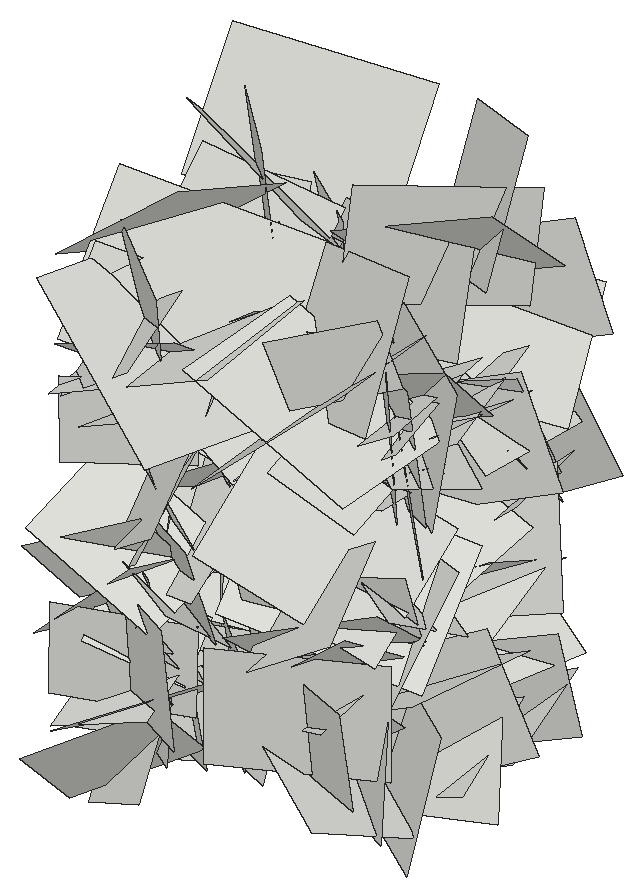
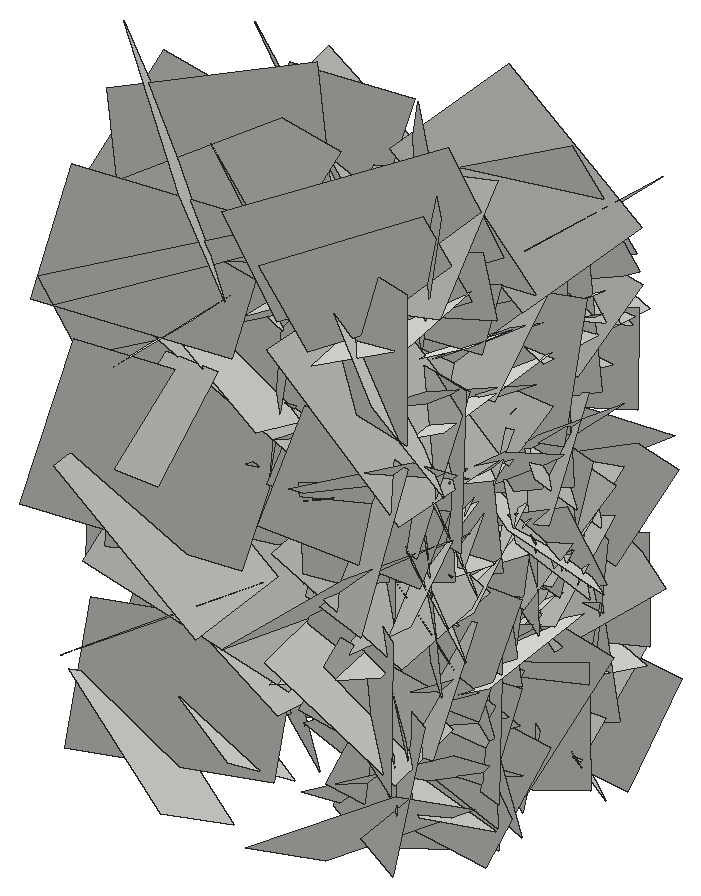
# SketchUp Ruby script. Lengths in inches.
U = 1.inch
M = Sketchup.active_model
def pt(a) = Geom::Point3d.new(a.map { |v| v * U })
def face(e, loops, mat)
  f = e.add_face(loops[0].map { |a| pt(a) })
  loops[1..].each { |l| e.add_face(l.map { |a| pt(a) }).erase! }
  f.material = f.back_material = mat if mat
  f
end
# faces: each face lists its corners as indices into pts; further lists are holes
def faces(e, pts, list, mat = nil) = list.each { |f| face(e, (f[0].is_a?(Array) ? f : [f]).map { |l| l.map { |i| pts[i] } }, mat) }
# xy, xz, yz: faces in a plane at the given z, y or x. An outline is a flat list of corners, or four numbers for a rectangle; further outlines are holes
def ring(l) = l.size == 4 ? [[l[0], l[1]], [l[2], l[1]], [l[2], l[3]], [l[0], l[3]]] : l.each_slice(2).to_a
def flat(e, list, mat, &to3) = list.each { |f| face(e, (f[0].is_a?(Array) ? f : [f]).map { |l| ring(l).map { |u, v| to3.(u, v) } }, mat) }
def xy(e, z, list, mat = nil) = flat(e, list, mat) { |x, y| [x, y, z] }
def xz(e, y, list, mat = nil) = flat(e, list, mat) { |x, z| [x, y, z] }
def yz(e, x, list, mat = nil) = flat(e, list, mat) { |y, z| [x, y, z] }
def lines(e, pts, list) = list.each { |a, b| e.add_line(pt(pts[a]), pt(pts[b])) }
# prism: a flat outline (further loops are holes) pulled along v
def prism(e, loops, v, mat = nil)
  f = face(e, loops, mat); d = Geom::Vector3d.new(v.map { |x| x * U })
  f.pushpull(f.normal.samedirection?(d) ? d.length : -d.length)
end
def box(e, o, s, mat = nil) = prism(e, [[o, [o[0] + s[0], o[1], o[2]], [o[0] + s[0], o[1] + s[1], o[2]], [o[0], o[1] + s[1], o[2]]]], [0, 0, s[2]], mat)
def at(x, y, z, deg = 0) = Geom::Transformation.translation(pt([x, y, z])) * Geom::Transformation.rotation(ORIGIN, Z_AXIS, deg.degrees)
def axes(o, x, y, z) = Geom::Transformation.new([*x, 0, *y, 0, *z, 0, *pt(o).to_a, 1])
def part(name) = M.definitions.add(name)
# library, detail: a bought-in or finely detailed component or shape, given as its bounding box
def library(name, o, s) = part(name).tap { |d| box(d.entities, o, s) }
def detail(e, o, s) = box(e.add_group.entities, o, s)
def put(e, d, t, mat = nil) = e.add_instance(d, t).tap { |i| i.material = mat if mat }
def group(e, t, mat = nil) = e.add_group.tap { |g| g.transformation = t; g.material = mat if mat }.entities
root = M.entities
c1 = part("Component\#6")
p = [[0.01,0,0],[0,3.24,4.54],[4.32,3.24,4.54],[4.33,0,0]]
faces(c1.entities,p,[[0,1,2,3]])
put(root,c1,axes([414.68,154.27,5.56],[0.10843,0.64197,-0.78685],[0.13439,-0.79271,-0.63027],[-1.06801,-0.03458,-0.15919]))
put(root,c1,axes([410.71,149.67,1.32],[0.10197,-0.47157,-0.58691],[-0.00963,-0.59236,0.47447],[0.798,0.05311,0.08072]))
put(root,c1,axes([410.71,151.77,10.3],[0.00621,-0.04081,-0.81439],[0.02737,-0.814,0.04098],[0.86391,0.02608,0.00455]))
put(root,c1,axes([414.68,158.76,13.54],[0.17018,-0.33172,-0.9968],[0.1229,-0.99662,0.35033],[-1.10678,-0.16167,-0.11436]))
put(root,c1,axes([410.71,155.14,21.07],[-0.01676,0.7943,-0.14622],[0.08914,-0.14383,-0.79043],[0.85145,0.03069,0.07988]))
put(root,c1,axes([414.68,152.55,8.85],[0.17208,0.39932,0.93109],[0.08126,0.93542,-0.41455],[-1.07081,0.13515,0.11817]))
put(root,c1,axes([410.71,155.22,14.18],[-0.0107,0.67836,0.43703],[0.08223,0.43585,-0.67474],[0.8514,-0.03357,0.07066]))
put(root,c1,axes([414.68,154.72,7.86],[-0.01434,-0.12328,-0.7123],[-0.10241,-0.70572,0.12398],[-0.75939,0.0975,-0.00327]))
put(root,c1,axes([410.71,153.88,7.81],[0.12498,-0.19712,-0.75186],[-0.05107,-0.76085,0.19192],[0.82232,-0.01729,0.12619]))
put(root,c1,axes([414.68,156.49,11.61],[0.16435,-0.92659,-0.48849],[0.14398,-0.47186,0.93815],[-1.10094,-0.20004,0.04977]))
put(root,c1,axes([414.68,155.82,10.86],[0.10869,-0.77244,0.23734],[-0.13092,0.22145,0.77409],[-0.8465,-0.13343,-0.08925]))
put(root,c1,axes([410.71,152.8,10.75],[-0.04843,-0.82009,-0.82841],[-0.32646,-0.79109,0.80013],[1.19171,-0.25004,0.18553]))
put(root,c1,axes([410.71,146.53,12.92],[0.03124,-0.05121,0.8385],[-0.00373,0.839,0.05136],[0.89046,0.00531,-0.0292]))
put(root,c1,axes([410.71,155.95,10.68],[0.04823,-0.00518,0.84226],[-0.02844,0.84305,0.00663],[0.89236,0.02715,-0.04531]))
put(root,c1,axes([414.68,154.86,6.54],[0.11481,0.21277,-0.79232],[-0.09254,-0.79167,-0.22453],[-0.86468,0.11298,-0.08117]))
put(root,c1,axes([410.71,147.06,-0.97],[0.01135,-0.66277,0.66685],[-0.09721,0.66298,0.66039],[0.99185,0.07256,0.05709]))
put(root,c1,axes([414.68,155.74,21.65],[0.00825,-0.17983,-0.66547],[-0.14401,-0.65286,0.17483],[-0.71636,0.12918,-0.04281]))
put(root,c1,axes([414.68,153.02,6.56],[-0.04835,0.51462,-0.41299],[-0.10228,-0.41473,-0.50612],[-0.69191,0.02534,0.10368]))
put(root,c1,axes([410.71,149.625,17.57],[0.05592,-0.7816,-0.40589],[-0.0657,-0.4089,0.77935],[0.93124,0.01809,0.07936]))
put(root,c1,axes([410.71,152.46,19.1],[-0.24316,-1.11668,0.32256],[-0.08367,0.34299,1.13127],[1.22923,-0.19755,0.14081]))
put(root,c1,axes([410.71,154.93,13.48],[-0.13332,0.92748,-0.67904],[-0.1887,-0.69057,-0.91025],[1.20375,-0.00553,-0.2179]))
put(root,c1,axes([414.68,155.23,10.47],[0.04155,0.12694,-0.87349],[0.11983,-0.86787,-0.12105],[-0.92792,-0.10639,-0.05475]))
put(root,c1,axes([410.71,153.68,-0.24],[0.08313,-0.05331,0.78078],[0.05564,0.78328,0.04821],[0.82769,-0.0473,-0.08166]))
put(root,c1,axes([414.68,152.53,7.1875],[-0.08757,-0.64703,0.3684],[0.09594,0.35919,0.65114],[-0.78338,0.11632,0.03856]))
put(root,c1,axes([414.68,154.48,3.89],[-0.11783,0.23417,0.69133],[0.11259,0.69704,-0.21902],[-0.76547,0.06648,-0.13863]))
put(root,c1,axes([410.71,151.57,3.27],[0.14157,0.02397,-0.74069],[0.04702,-0.75154,-0.01632],[0.78414,0.04073,0.1347]))
put(root,c1,axes([414.68,146.09,12.1875],[0.18427,0.52878,-0.65011],[-0.11203,-0.64482,-0.55274],[-0.8812,0.19255,-0.06567]))
put(root,c1,axes([410.71,147.21,13.43],[-0.06341,1.09172,0.23851],[-0.19798,0.22572,-1.08003],[1.16785,0.09755,-0.17015]))
put(root,c1,axes([414.68,145.53,10.42],[0.22479,1.04725,-0.16356],[0.16331,-0.19548,-1.05191],[-1.11161,0.18306,-0.18761]))
put(root,c1,axes([410.71,149.03,14.67],[-0.12882,0.64149,-0.81464],[0.00451,-0.8199,-0.64626],[1.09909,0.07855,-0.09282]))
put(root,c1,axes([414.68,155.43,2.74],[-0.05213,0.12024,0.7107],[0.06472,0.71048,-0.11598],[-0.7613,0.05216,-0.05853]))
put(root,c1,axes([410.71,146.38,17.95],[0.09245,0.38694,0.78979],[-0.04684,0.79459,-0.38441],[0.93107,0.00155,-0.09776]))
put(root,c1,axes([414.68,155.07,5.6],[0.26442,-0.95782,0.42161],[0.12666,0.45666,0.96674],[-1.10204,-0.17733,0.21227]))
put(root,c1,axes([414.68,154.81,5.31],[-0.03271,-0.68931,-0.29186],[0.0897,-0.29345,0.68411],[-0.78838,-0.00479,0.08995]))
put(root,c1,axes([414.68,148.44,10.1],[-0.02371,0.59128,0.15103],[-0.13632,0.14317,-0.57956],[-0.63236,-0.05303,0.11928]))
put(root,c1,axes([410.71,154.73,4.99],[-0.23466,-0.21907,1.02966],[0.17179,1.03255,0.25453],[1.10257,-0.20751,0.17949]))
put(root,c1,axes([410.71,152.28,1.18],[-0.22482,-0.75958,0.923],[-0.06114,0.94282,0.76264],[1.2656,-0.08938,0.2008]))
put(root,c1,axes([414.68,146.72,8.375],[-0.05548,0.31048,0.67068],[0.12303,0.66747,-0.29994],[-0.77368,0.08387,-0.09579]))
put(root,c1,axes([410.71,147.71,9.53],[-0.0202,0.73421,-0.62443],[0.01239,-0.62433,-0.73445],[1.02159,0.02209,-0.00344]))
put(root,c1,axes([414.68,148.39,13.69],[-0.056,0.56116,0.2115],[-0.06403,0.20626,-0.56234],[-0.63244,-0.07057,0.03821]))
put(root,c1,axes([410.71,149.64,15.49],[-0.05397,-0.71515,0.49033],[0.26351,0.45852,0.69456],[0.88054,-0.18105,-0.1778]))
put(root,c1,axes([410.71,157.06,14.03],[-0.04606,-0.47436,-0.98882],[-0.12961,-0.98133,0.47614],[1.15527,-0.12901,0.01399]))
put(root,c1,axes([410.71,159.16,9.85],[-0.13765,0.1916,-1.18129],[-0.14512,-1.1828,-0.17679],[1.2602,-0.11528,-0.14939]))
put(root,c1,axes([410.71,152.91,14.99],[-0.05042,0.65822,-0.8803],[-0.11398,-0.87969,-0.65195],[1.15954,-0.05785,-0.10236]))
put(root,c1,axes([410.71,158.68,8.63],[-0.07829,-0.94373,0.27717],[0.10215,0.26967,0.94388],[1.03759,-0.09775,-0.07202]))
put(root,c1,axes([414.68,147.13,6.96],[0.04816,-0.19283,0.63159],[-0.07038,0.62854,0.19668],[-0.69645,-0.07685,0.0238]))
put(root,c1,axes([410.71,152.6,3.91],[0.02426,0.68313,0.69515],[-0.0107,0.69547,-0.68312],[1.03305,-0.00884,-0.0234]))
put(root,c1,axes([414.68,153.92,20.8125],[-0.01755,0.277,-0.54123],[-0.05617,-0.54003,-0.27476],[-0.64202,0.03967,0.03883]))
put(root,c1,axes([414.68,156.87,7.65],[-0.00449,0.50233,-0.39291],[-0.02578,-0.39276,-0.50188],[-0.67552,0.01165,0.02176]))
put(root,c1,axes([414.68,147.62,1.41],[0.08717,-0.06025,0.7019],[-0.04865,0.70471,0.06586],[-0.74517,-0.05306,0.07781]))
put(root,c1,axes([414.68,151.79,4.27],[0.00282,-0.67031,0.14172],[0.04158,0.14164,0.66918],[-0.72504,0.00552,0.03892]))
put(root,c1,axes([414.68,151.99,2.12],[0.1775,0.68354,0.35821],[-0.06031,0.37649,-0.69181],[-0.81579,0.12089,0.12909]))
put(root,c1,axes([410.71,154.79,8.7],[-0.06507,0.61236,-0.89404],[-0.03144,-0.89608,-0.61173],[1.14823,0.01016,-0.06741]))
put(root,c1,axes([410.71,155.05,20.66],[0.11898,0.43702,0.87755],[-0.10329,0.88388,-0.42771],[1.03402,0.038,-0.1437]))
put(root,c1,axes([410.71,148.76,4.0625],[0.10183,-0.75916,-0.2873],[0.20096,-0.26032,0.75126],[0.83661,0.15493,-0.14549]))
put(root,c1,axes([414.68,151.13,9.12],[0.15296,0.67587,0.31221],[-0.03502,0.32352,-0.68509],[-0.78839,0.11676,0.09101]))
put(root,c1,axes([410.71,158.45,22.43],[-0.19892,0.24365,-1.12098],[0.08242,-1.13056,-0.25875],[1.21318,0.11676,-0.16622]))
put(root,c1,axes([410.71,153.47,7.93],[-0.25077,0.36385,-1.26635],[-0.08689,-1.28818,-0.35481],[1.39394,-0.01484,-0.24993]))
put(root,c1,axes([414.68,151.91,13.09],[0.06029,-0.61389,0.14039],[-0.0496,0.13645,0.61563],[-0.66568,-0.06576,-0.03315]))
put(root,c1,axes([414.68,155.37,8.05],[0.03179,-0.04018,0.69029],[0.07893,0.6871,0.03676],[-0.72868,0.07267,0.03409]))
put(root,c1,axes([414.68,147.25,18.09],[0.11506,-0.20062,0.68841],[0.02156,0.69683,0.19986],[-0.75976,-0.01061,0.10993]))
put(root,c1,axes([414.68,146,16.15],[0.10062,0.63244,0.10884],[-0.07256,0.11937,-0.63396],[-0.67636,0.08128,0.0842]))
put(root,c1,axes([410.71,157.74,11.21],[0.0595,-0.6331,0.72554],[0.06262,0.72766,0.63038],[1.01877,-0.00775,-0.08112]))
put(root,c1,axes([410.71,160.22,19.0625],[-0.13961,-0.68099,-1.03193],[-0.07146,-1.03227,0.68982],[1.30861,-0.12902,-0.07242]))
put(root,c1,axes([414.68,149.02,5.32],[0.19432,-0.67994,0.40742],[0.04988,0.42677,0.69106],[-0.83874,-0.13215,0.13549]))
put(root,c1,axes([410.71,154.9,1.8],[0.03269,0.90387,0.50014],[0.00572,0.50021,-0.90434],[1.09498,-0.0296,-0.01021]))
put(root,c1,axes([414.68,152.72,13.34],[0.14332,-0.62648,-0.12325],[-0.10799,-0.14554,0.62801],[-0.66813,-0.11086,-0.12794]))
put(root,c1,axes([410.71,157.43,12.97],[-0.1074,-0.05602,-1.35571],[-0.22854,-1.34155,0.07155],[1.42001,-0.22014,-0.09102]))
put(root,c1,axes([410.71,151.01,19.39],[0.01021,0.65154,-0.69294],[0.23408,-0.67557,-0.63214],[0.98066,0.15447,0.1581]))
put(root,c1,axes([410.71,148.31,17.26],[0.09379,0.98835,0.28145],[-0.01751,0.28383,-0.99149],[1.08916,-0.08054,-0.04018]))
put(root,c1,axes([410.71,155.4,17.52],[-0.19723,0.3027,-1.19403],[0.0763,-1.20284,-0.31615],[1.30348,0.11621,-0.16216]))
put(root,c1,axes([410.71,145.87,3.84],[0.08046,-0.07863,0.91675],[0.19442,0.90269,0.06223],[0.95574,-0.17701,-0.08983]))
put(root,c1,axes([410.71,148.09,7.11],[-0.15706,0.67864,1.02073],[0.03183,1.02986,-0.68036],[1.29889,0.05683,0.1401]))
put(root,c1,axes([410.71,148.93,-0.125],[-0.17085,0.2332,1.25619],[-0.02467,1.2654,-0.2379],[1.35409,0.05247,0.15416]))
put(root,c1,axes([410.71,158.83,13.98],[0.00743,-1.2386,0.03478],[-0.17851,0.0335,1.22715],[1.30124,0.01167,0.16814]))
put(root,c1,axes([410.71,152.08,1.74],[0.04493,0.85391,0.54577],[0.09586,0.54089,-0.85328],[1.06994,-0.08432,0.05353]))
put(root,c1,axes([410.71,151.75,19.45],[0.16935,0.44212,0.83371],[0.05466,0.84022,-0.45546],[0.99881,-0.12095,-0.11643]))
put(root,c1,axes([414.68,150.18,6.375],[0.17639,-0.58204,-0.33942],[-0.00316,-0.35025,0.59915],[-0.71419,-0.1422,-0.08648]))
put(root,c1,axes([414.68,148.65,3.04],[0.12439,-0.47488,0.46679],[0.05284,0.47892,0.47469],[-0.70386,-0.04797,0.11813]))
put(root,c1,axes([410.71,156.6875,24.44],[0.16473,0.01802,-1.18121],[-0.23771,-1.16927,-0.04735],[1.22945,-0.22849,0.14911]))
put(root,c1,axes([410.71,147.43,1.76],[0.0449,0.15818,1.07958],[0.0304,1.07985,-0.15935],[1.15617,-0.03454,-0.03773]))
put(root,c1,axes([410.71,158.38,15.93],[-0.03304,0.59909,-1.16183],[-0.1621,-1.15585,-0.5919],[1.37611,-0.12177,-0.09762]))
put(root,c1,axes([410.71,156.09,10.89],[0.02844,-1.01096,-0.23497],[0.17327,-0.228,0.99963],[1.08645,0.06282,-0.15327]))
put(root,c1,axes([410.71,159.05,4.5],[0.22831,-0.97739,-0.02602],[-0.01319,-0.02938,1.00067],[1.03632,0.21495,0.01847]))
put(root,c1,axes([410.71,157.5,5.99],[0.02733,0.34478,-1.12821],[-0.04378,-1.12752,-0.34552],[1.24973,-0.04704,0.01257]))
put(root,c1,axes([410.71,147.25,11.15],[0.01251,0.83252,-0.66438],[0.16644,-0.65852,-0.82239],[1.1167,0.08883,0.13002]))
put(root,c1,axes([410.71,153.16,13.74],[0.07693,-1.07175,0.44962],[-0.07215,0.4458,1.07364],[1.22986,0.09319,0.03486]))
put(root,c1,axes([410.71,150.33,13.2],[-0.24126,0.02501,1.36725],[0.05252,1.3853,-0.01709],[1.44858,-0.04606,0.22834]))
put(root,c1,axes([410.71,144.59,11.1],[0.20686,0.83944,0.54314],[0.00436,0.55271,-0.85571],[1.05982,-0.16612,-0.10249]))
put(root,c1,axes([410.71,153.72,24.55],[-0.10736,0.8301,-0.78481],[0.26067,-0.75358,-0.8288],[1.18252,0.24148,0.11144]))
put(root,c1,axes([410.71,148.8125,12.02],[0.02959,0.36254,-1.01381],[0.21176,-0.99828,-0.35148],[1.12146,0.17893,0.09312]))
put(root,c1,axes([410.71,148.37,14.37],[0.13394,0.02599,1.3483],[-0.3112,1.32226,0.00203],[1.39518,0.29244,-0.12899]))
put(root,c1,axes([410.71,151.84,12.71],[0.09641,-0.969,-0.91768],[-0.24854,-0.9171,0.94515],[1.39265,-0.09659,0.2322]))
put(root,c1,axes([410.71,152.41,8.09],[-0.02535,-1.06677,0.60381],[0.0625,0.60222,1.06631],[1.29785,-0.04984,-0.03955]))
put(root,c1,axes([410.71,153.41,21.56],[0.04666,0.60871,1.19242],[-0.17987,1.18598,-0.59916],[1.40769,0.13136,-0.11609]))
put(root,c1,axes([410.71,154.4,5.48],[-0.14525,-0.2612,-1.20099],[0.27145,-1.18798,0.22915],[1.27422,0.2233,-0.18571]))
put(root,c1,axes([410.71,148.05,8.79],[0.07068,0.0827,-1.14811],[0.1221,-1.14474,-0.07576],[1.21402,0.11031,0.07447]))
put(root,c1,axes([410.71,153.21,11.43],[-0.14123,-0.96535,-0.93141],[0.15435,-0.94087,0.95433],[1.41351,0.00629,-0.19727]))
put(root,c1,axes([410.71,157.09,9.16],[0.26081,-0.66319,-0.77037],[0.09697,-0.77495,0.69635],[1.07312,0.23121,0.12431]))
put(root,c1,axes([410.71,149.27,6.59],[-0.15688,1.33929,-0.00269],[0.18956,0.01708,-1.33541],[1.40693,0.14704,0.17962]))
put(root,c1,axes([410.71,149.82,11.51],[0.16938,-0.10345,1.35904],[-0.25816,1.34416,0.13095],[1.4215,0.25644,-0.13816]))
put(root,c1,axes([410.71,155.16,12.125],[0.20792,1.23942,0.0793],[-0.14973,0.10203,-1.24521],[1.30793,-0.18535,-0.15516]))
put(root,c1,axes([410.71,151.77,16.16],[0.14743,1.12249,0.38129],[0.0578,0.37744,-1.13105],[1.25528,-0.14922,0.00729]))
put(root,c1,axes([410.71,145.22,20.96],[0.20751,1.35949,-0.09859],[-0.20583,-0.07077,-1.36145],[1.43011,-0.20745,-0.18164]))
put(root,c1,axes([410.71,149.47,1.18],[0.22795,-1.08393,0.44752],[0.03192,0.45993,1.09954],[1.24263,0.18702,-0.11034]))
put(root,c1,axes([410.71,155.15,17.37],[0.02517,0.60882,-1.16754],[0.2041,-1.15679,-0.59929],[1.38075,0.1599,0.10987]))
put(root,c1,axes([410.71,146.56,18.67],[0.08115,0.67304,1.19325],[0.03541,1.19384,-0.67552],[1.45175,-0.06674,-0.05023]))
put(root,c1,axes([410.71,150.46,17.01],[0.04698,1.34267,-0.16756],[0.13374,-0.17102,-1.33703],[1.42802,-0.02815,0.13073]))
put(root,c1,axes([410.71,150.02,13.53],[0.11354,-0.10924,1.28227],[0.18202,1.27641,0.09439],[1.35193,-0.16268,-0.1204]))
put(root,c1,axes([410.71,153.54,10.59],[0.17173,1.22834,-0.55665],[0.01226,-0.5619,-1.23655],[1.42944,-0.14275,0.07748]))
put(root,c1,axes([410.71,151.36,16.73],[0.05564,-1.33407,-0.12972],[0.26745,-0.11766,1.31218],[1.39538,0.07575,-0.24633]))
put(root,c1,axes([410.71,148.21,18.05],[0.18781,1.38239,0.05917],[0.11095,0.04609,-1.39025],[1.46247,-0.18102,0.09787]))
put(root,c1,axes([424.49,148.21,18.05],[-0.18781,1.38239,0.05917],[-0.11095,0.04609,-1.39025],[-1.46247,-0.18102,0.09787]))
put(root,c1,axes([424.49,151.36,16.73],[-0.05564,-1.33407,-0.12972],[-0.26745,-0.11766,1.31218],[-1.39538,0.07575,-0.24633]))
put(root,c1,axes([424.49,153.54,10.59],[-0.17173,1.22834,-0.55665],[-0.01226,-0.5619,-1.23655],[-1.42944,-0.14275,0.07748]))
put(root,c1,axes([424.49,150.02,13.53],[-0.11354,-0.10924,1.28227],[-0.18202,1.27641,0.09439],[-1.35193,-0.16268,-0.1204]))
put(root,c1,axes([424.49,150.46,17.01],[-0.04698,1.34267,-0.16756],[-0.13374,-0.17102,-1.33703],[-1.42802,-0.02815,0.13073]))
put(root,c1,axes([424.49,146.56,18.67],[-0.08115,0.67304,1.19325],[-0.03541,1.19384,-0.67552],[-1.45175,-0.06674,-0.05023]))
put(root,c1,axes([424.49,155.15,17.37],[-0.02517,0.60882,-1.16754],[-0.2041,-1.15679,-0.59929],[-1.38075,0.1599,0.10987]))
put(root,c1,axes([424.49,149.47,1.18],[-0.22795,-1.08393,0.44752],[-0.03192,0.45993,1.09954],[-1.24263,0.18702,-0.11034]))
put(root,c1,axes([424.49,145.22,20.96],[-0.20751,1.35949,-0.09859],[0.20583,-0.07077,-1.36145],[-1.43011,-0.20745,-0.18164]))
put(root,c1,axes([424.49,151.77,16.16],[-0.14743,1.12249,0.38129],[-0.0578,0.37744,-1.13105],[-1.25528,-0.14922,0.00729]))
put(root,c1,axes([424.49,155.16,12.125],[-0.20792,1.23942,0.0793],[0.14973,0.10203,-1.24521],[-1.30793,-0.18535,-0.15516]))
put(root,c1,axes([424.49,149.82,11.51],[-0.16938,-0.10345,1.35904],[0.25816,1.34416,0.13095],[-1.4215,0.25644,-0.13816]))
put(root,c1,axes([424.49,149.27,6.59],[0.15688,1.33929,-0.00269],[-0.18956,0.01708,-1.33541],[-1.40693,0.14704,0.17962]))
put(root,c1,axes([424.49,157.09,9.16],[-0.26081,-0.66319,-0.77037],[-0.09697,-0.77495,0.69635],[-1.07312,0.23121,0.12431]))
put(root,c1,axes([424.49,153.21,11.43],[0.14123,-0.96535,-0.93141],[-0.15435,-0.94087,0.95433],[-1.41351,0.00629,-0.19727]))
put(root,c1,axes([424.49,148.05,8.79],[-0.07068,0.0827,-1.14811],[-0.1221,-1.14474,-0.07576],[-1.21402,0.11031,0.07447]))
put(root,c1,axes([424.49,154.4,5.48],[0.14525,-0.2612,-1.20099],[-0.27145,-1.18798,0.22915],[-1.27422,0.2233,-0.18571]))
put(root,c1,axes([424.49,153.41,21.56],[-0.04666,0.60871,1.19242],[0.17987,1.18598,-0.59916],[-1.40769,0.13136,-0.11609]))
put(root,c1,axes([424.49,152.41,8.09],[0.02535,-1.06677,0.60381],[-0.0625,0.60222,1.06631],[-1.29785,-0.04984,-0.03955]))
put(root,c1,axes([424.49,151.84,12.71],[-0.09641,-0.969,-0.91768],[0.24854,-0.9171,0.94515],[-1.39265,-0.09659,0.2322]))
put(root,c1,axes([424.49,148.37,14.37],[-0.13394,0.02599,1.3483],[0.3112,1.32226,0.00203],[-1.39518,0.29244,-0.12899]))
put(root,c1,axes([424.49,148.8125,12.02],[-0.02959,0.36254,-1.01381],[-0.21176,-0.99828,-0.35148],[-1.12146,0.17893,0.09312]))
put(root,c1,axes([424.49,153.72,24.55],[0.10736,0.8301,-0.78481],[-0.26067,-0.75358,-0.8288],[-1.18252,0.24148,0.11144]))
put(root,c1,axes([424.49,144.59,11.1],[-0.20686,0.83944,0.54314],[-0.00436,0.55271,-0.85571],[-1.05982,-0.16612,-0.10249]))
put(root,c1,axes([424.49,150.33,13.2],[0.24126,0.02501,1.36725],[-0.05252,1.3853,-0.01709],[-1.44858,-0.04606,0.22834]))
put(root,c1,axes([424.49,153.16,13.74],[-0.07693,-1.07175,0.44962],[0.07215,0.4458,1.07364],[-1.22986,0.09319,0.03486]))
put(root,c1,axes([424.49,147.25,11.15],[-0.01251,0.83252,-0.66438],[-0.16644,-0.65852,-0.82239],[-1.1167,0.08883,0.13002]))
put(root,c1,axes([424.49,157.5,5.99],[-0.02733,0.34478,-1.12821],[0.04378,-1.12752,-0.34552],[-1.24973,-0.04704,0.01257]))
put(root,c1,axes([424.49,159.05,4.5],[-0.22831,-0.97739,-0.02602],[0.01319,-0.02938,1.00067],[-1.03632,0.21495,0.01847]))
put(root,c1,axes([424.49,156.09,10.89],[-0.02844,-1.01096,-0.23497],[-0.17327,-0.228,0.99963],[-1.08645,0.06282,-0.15327]))
put(root,c1,axes([424.49,158.38,15.93],[0.03304,0.59909,-1.16183],[0.1621,-1.15585,-0.5919],[-1.37611,-0.12177,-0.09762]))
put(root,c1,axes([424.49,147.43,1.76],[-0.0449,0.15818,1.07958],[-0.0304,1.07985,-0.15935],[-1.15617,-0.03454,-0.03773]))
put(root,c1,axes([424.49,156.6875,24.44],[-0.16473,0.01802,-1.18121],[0.23771,-1.16927,-0.04735],[-1.22945,-0.22849,0.14911]))
put(root,c1,axes([420.52,148.65,3.04],[-0.12439,-0.47488,0.46679],[-0.05284,0.47892,0.47469],[0.70386,-0.04797,0.11813]))
put(root,c1,axes([420.52,150.18,6.375],[-0.17639,-0.58204,-0.33942],[0.00316,-0.35025,0.59915],[0.71419,-0.1422,-0.08648]))
put(root,c1,axes([424.49,151.75,19.45],[-0.16935,0.44212,0.83371],[-0.05466,0.84022,-0.45546],[-0.99881,-0.12095,-0.11643]))
put(root,c1,axes([424.49,152.08,1.74],[-0.04493,0.85391,0.54577],[-0.09586,0.54089,-0.85328],[-1.06994,-0.08432,0.05353]))
put(root,c1,axes([424.49,158.83,13.98],[-0.00743,-1.2386,0.03478],[0.17851,0.0335,1.22715],[-1.30124,0.01167,0.16814]))
put(root,c1,axes([424.49,148.93,-0.125],[0.17085,0.2332,1.25619],[0.02467,1.2654,-0.2379],[-1.35409,0.05247,0.15416]))
put(root,c1,axes([424.49,148.09,7.11],[0.15706,0.67864,1.02073],[-0.03183,1.02986,-0.68036],[-1.29889,0.05683,0.1401]))
put(root,c1,axes([424.49,145.87,3.84],[-0.08046,-0.07863,0.91675],[-0.19442,0.90269,0.06223],[-0.95574,-0.17701,-0.08983]))
put(root,c1,axes([424.49,155.4,17.52],[0.19723,0.3027,-1.19403],[-0.0763,-1.20284,-0.31615],[-1.30348,0.11621,-0.16216]))
put(root,c1,axes([424.49,148.31,17.26],[-0.09379,0.98835,0.28145],[0.01751,0.28383,-0.99149],[-1.08916,-0.08054,-0.04018]))
put(root,c1,axes([424.49,151.01,19.39],[-0.01021,0.65154,-0.69294],[-0.23408,-0.67557,-0.63214],[-0.98066,0.15447,0.1581]))
put(root,c1,axes([424.49,157.43,12.97],[0.1074,-0.05602,-1.35571],[0.22854,-1.34155,0.07155],[-1.42001,-0.22014,-0.09102]))
put(root,c1,axes([420.52,152.72,13.34],[-0.14332,-0.62648,-0.12325],[0.10799,-0.14554,0.62801],[0.66813,-0.11086,-0.12794]))
put(root,c1,axes([424.49,154.9,1.8],[-0.03269,0.90387,0.50014],[-0.00572,0.50021,-0.90434],[-1.09498,-0.0296,-0.01021]))
put(root,c1,axes([420.52,149.02,5.32],[-0.19432,-0.67994,0.40742],[-0.04988,0.42677,0.69106],[0.83874,-0.13215,0.13549]))
put(root,c1,axes([424.49,160.22,19.0625],[0.13961,-0.68099,-1.03193],[0.07146,-1.03227,0.68982],[-1.30861,-0.12902,-0.07242]))
put(root,c1,axes([424.49,157.74,11.21],[-0.0595,-0.6331,0.72554],[-0.06262,0.72766,0.63038],[-1.01877,-0.00775,-0.08112]))
put(root,c1,axes([420.52,146,16.15],[-0.10062,0.63244,0.10884],[0.07256,0.11937,-0.63396],[0.67636,0.08128,0.0842]))
put(root,c1,axes([420.52,147.25,18.09],[-0.11506,-0.20062,0.68841],[-0.02156,0.69683,0.19986],[0.75976,-0.01061,0.10993]))
put(root,c1,axes([420.52,155.37,8.05],[-0.03179,-0.04018,0.69029],[-0.07893,0.6871,0.03676],[0.72868,0.07267,0.03409]))
put(root,c1,axes([420.52,151.91,13.09],[-0.06029,-0.61389,0.14039],[0.0496,0.13645,0.61563],[0.66568,-0.06576,-0.03315]))
put(root,c1,axes([424.49,153.47,7.93],[0.25077,0.36385,-1.26635],[0.08689,-1.28818,-0.35481],[-1.39394,-0.01484,-0.24993]))
put(root,c1,axes([424.49,158.45,22.43],[0.19892,0.24365,-1.12098],[-0.08242,-1.13056,-0.25875],[-1.21318,0.11676,-0.16622]))
